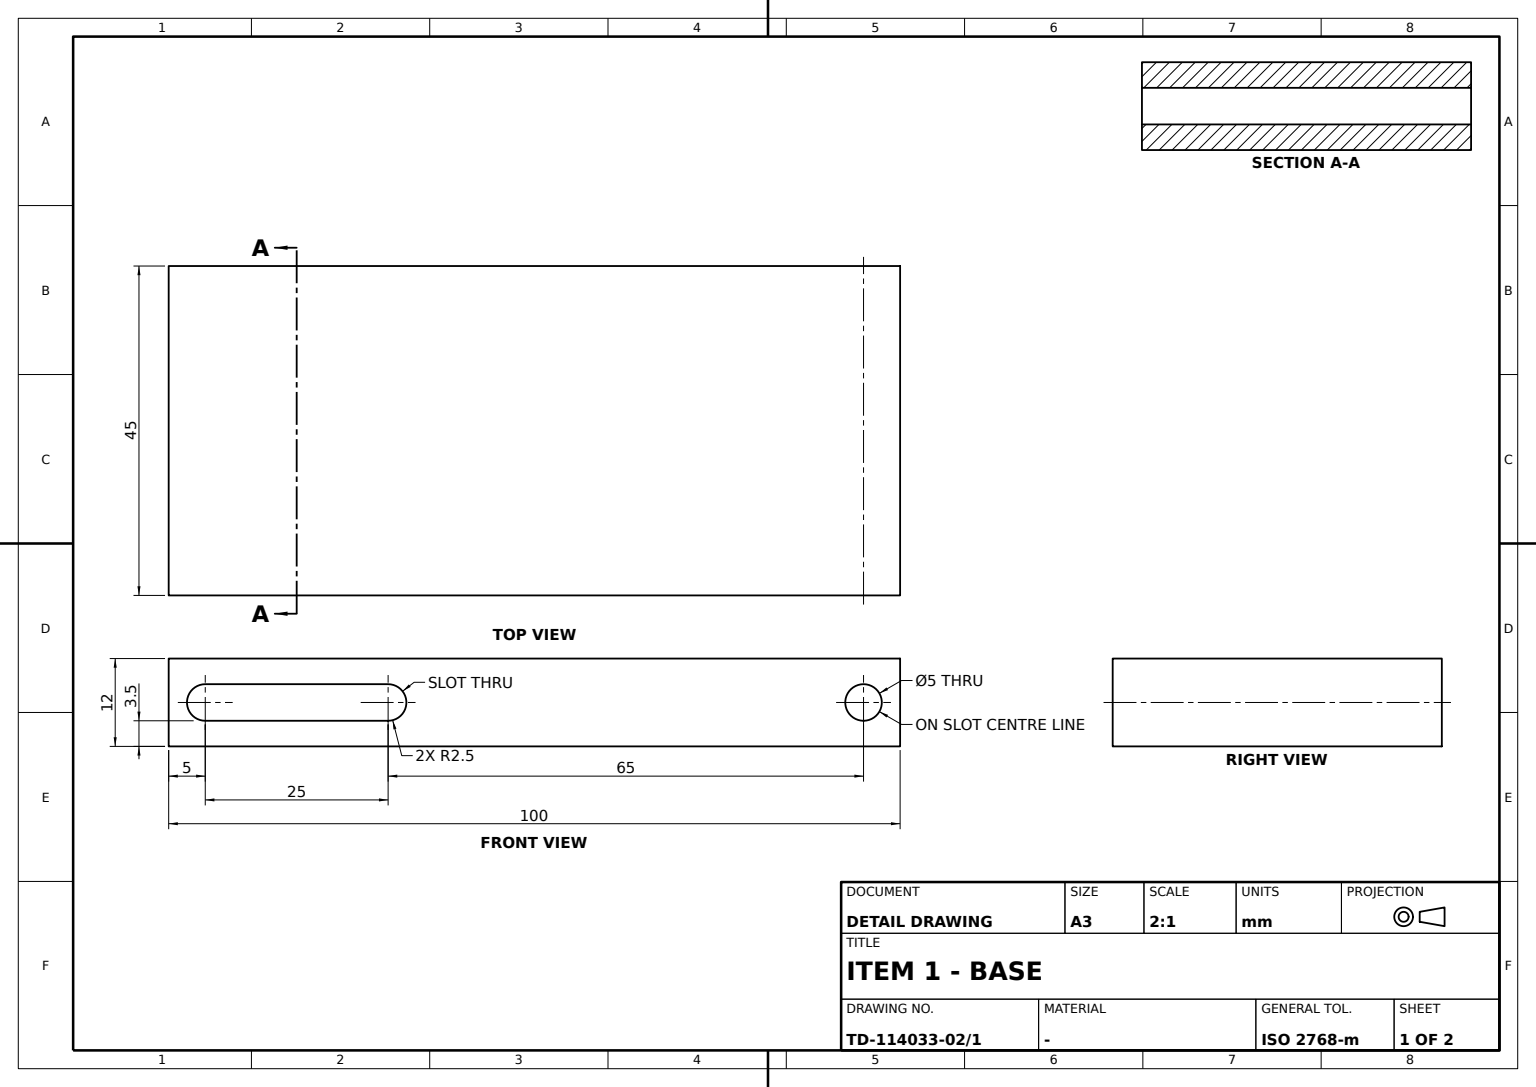
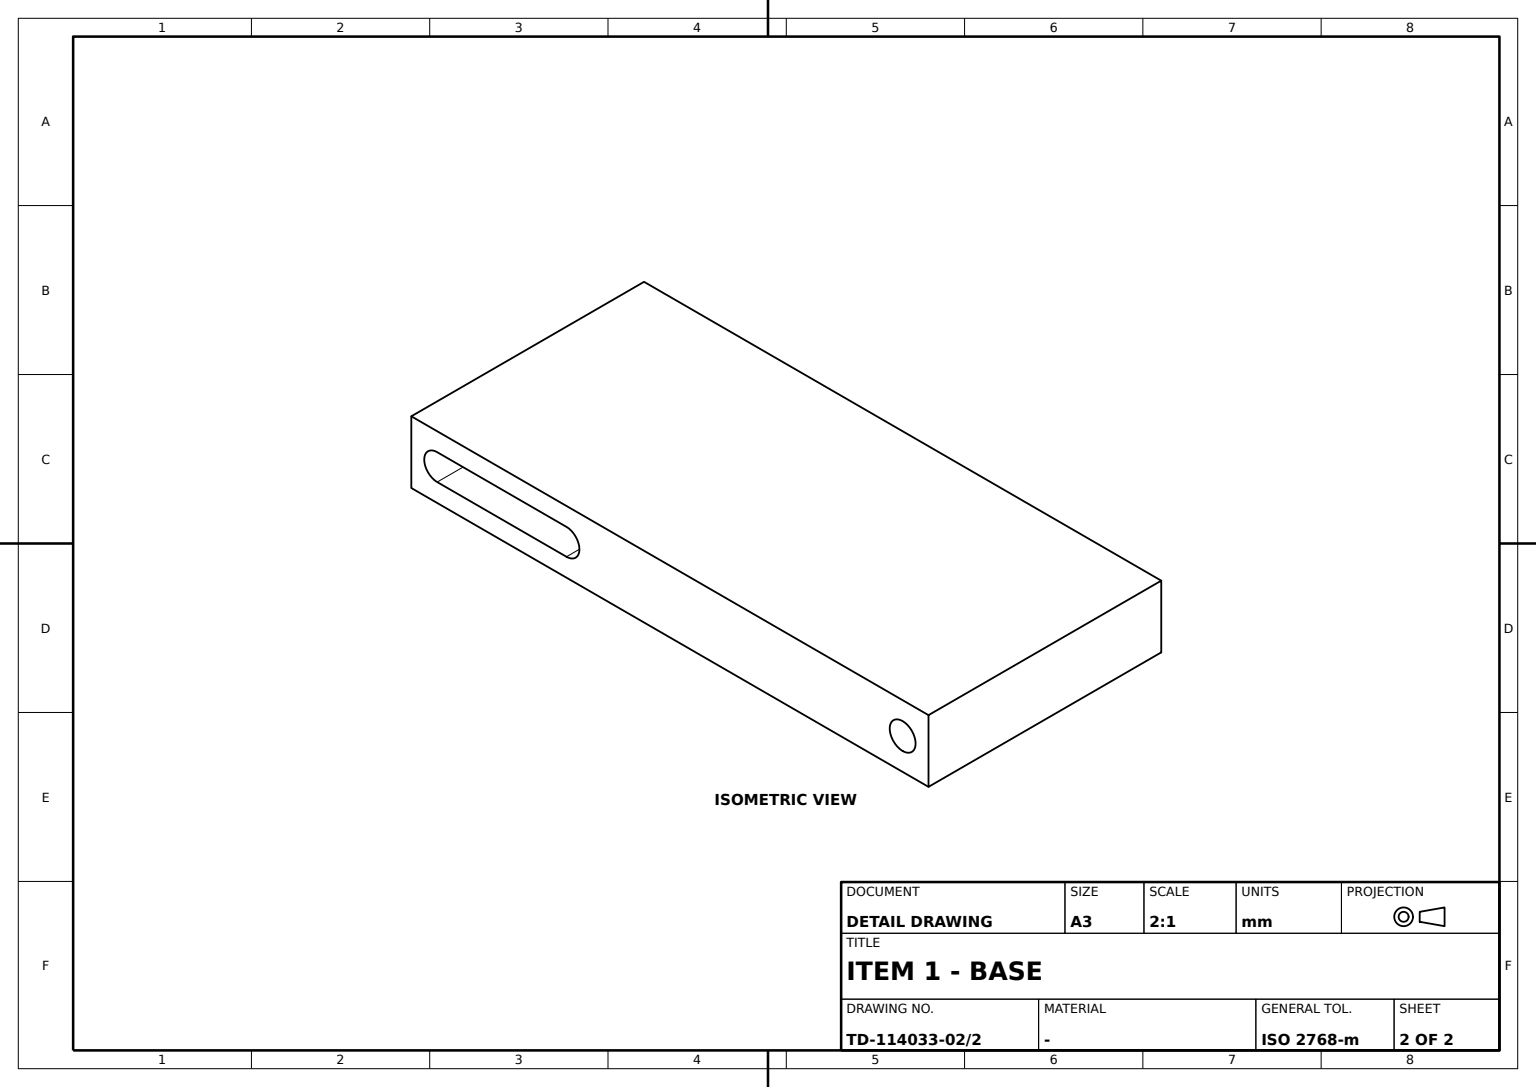
ISO-10303-21;
HEADER;
FILE_DESCRIPTION((''),'2;1');
FILE_NAME('','',(''),(''),'','','');
FILE_SCHEMA(('AUTOMOTIVE_DESIGN'));
ENDSEC;
DATA;
#1=APPLICATION_CONTEXT('');
#2=PRODUCT_CONTEXT('',#1,'mechanical');
#3=PRODUCT('','','',(#2));
#4=PRODUCT_DEFINITION_FORMATION('','',#3);
#5=PRODUCT_DEFINITION_CONTEXT('',#1,'design');
#6=PRODUCT_DEFINITION('','',#4,#5);
#7=PRODUCT_DEFINITION_SHAPE('','',#6);
#8=(LENGTH_UNIT()NAMED_UNIT(*)SI_UNIT(.MILLI.,.METRE.));
#9=(NAMED_UNIT(*)PLANE_ANGLE_UNIT()SI_UNIT($,.RADIAN.));
#10=(NAMED_UNIT(*)SI_UNIT($,.STERADIAN.)SOLID_ANGLE_UNIT());
#11=UNCERTAINTY_MEASURE_WITH_UNIT(LENGTH_MEASURE(0.005),#8,'distance_accuracy_value','');
#12=(GEOMETRIC_REPRESENTATION_CONTEXT(3)GLOBAL_UNCERTAINTY_ASSIGNED_CONTEXT((#11))GLOBAL_UNIT_ASSIGNED_CONTEXT((#8,#9,#10))REPRESENTATION_CONTEXT('',''));
#13=CARTESIAN_POINT('',(22.5,-20.,-2.5));
#14=VERTEX_POINT('',#13);
#15=CARTESIAN_POINT('',(22.5,-45.,-2.5));
#16=VERTEX_POINT('',#15);
#17=DIRECTION('',(0.,-1.,0.));
#18=VECTOR('',#17,1000.);
#19=LINE('',#13,#18);
#20=EDGE_CURVE('',#14,#16,#19,.T.);
#21=ORIENTED_EDGE('',*,*,#20,.F.);
#22=CARTESIAN_POINT('',(-22.5,-20.,-2.5));
#23=VERTEX_POINT('',#22);
#24=CARTESIAN_POINT('',(-0.66,-20.,-2.5));
#25=DIRECTION('',(1.,0.,0.));
#26=VECTOR('',#25,1000.);
#27=LINE('',#24,#26);
#28=EDGE_CURVE('',#14,#23,#27,.F.);
#29=ORIENTED_EDGE('',*,*,#28,.T.);
#30=CARTESIAN_POINT('',(-22.5,-45.,-2.5));
#31=VERTEX_POINT('',#30);
#32=LINE('',#22,#18);
#33=EDGE_CURVE('',#23,#31,#32,.T.);
#34=ORIENTED_EDGE('',*,*,#33,.T.);
#35=CARTESIAN_POINT('',(-0.66,-45.,-2.5));
#36=LINE('',#35,#26);
#37=EDGE_CURVE('',#16,#31,#36,.F.);
#38=ORIENTED_EDGE('',*,*,#37,.F.);
#39=EDGE_LOOP('',(#21,#29,#34,#38));
#40=FACE_BOUND('',#39,.T.);
#41=DIRECTION('',(0.,0.,-1.));
#42=AXIS2_PLACEMENT_3D('',#13,#41,#17);
#43=PLANE('',#42);
#44=ADVANCED_FACE('',(#40),#43,.F.);
#45=CARTESIAN_POINT('',(-22.5,50.,6.));
#46=VERTEX_POINT('',#45);
#47=CARTESIAN_POINT('',(-22.5,50.,-6.));
#48=VERTEX_POINT('',#47);
#49=CARTESIAN_POINT('',(-22.5,50.,0.));
#50=VECTOR('',#41,1000.);
#51=LINE('',#49,#50);
#52=EDGE_CURVE('',#46,#48,#51,.T.);
#53=ORIENTED_EDGE('',*,*,#52,.F.);
#54=CARTESIAN_POINT('',(22.5,50.,6.));
#55=VERTEX_POINT('',#54);
#56=CARTESIAN_POINT('',(0.,50.,6.));
#57=LINE('',#56,#26);
#58=EDGE_CURVE('',#46,#55,#57,.T.);
#59=ORIENTED_EDGE('',*,*,#58,.T.);
#60=CARTESIAN_POINT('',(22.5,50.,-6.));
#61=VERTEX_POINT('',#60);
#62=CARTESIAN_POINT('',(22.5,50.,0.));
#63=LINE('',#62,#50);
#64=EDGE_CURVE('',#55,#61,#63,.T.);
#65=ORIENTED_EDGE('',*,*,#64,.T.);
#66=CARTESIAN_POINT('',(0.,50.,-6.));
#67=LINE('',#66,#26);
#68=EDGE_CURVE('',#48,#61,#67,.T.);
#69=ORIENTED_EDGE('',*,*,#68,.F.);
#70=EDGE_LOOP('',(#53,#59,#65,#69));
#71=FACE_BOUND('',#70,.T.);
#72=AXIS2_PLACEMENT_3D('',#56,#17,#41);
#73=PLANE('',#72);
#74=ADVANCED_FACE('',(#71),#73,.F.);
#75=CARTESIAN_POINT('',(-22.5,-50.,6.));
#76=VERTEX_POINT('',#75);
#77=CARTESIAN_POINT('',(22.5,-50.,6.));
#78=VERTEX_POINT('',#77);
#79=CARTESIAN_POINT('',(0.,-50.,6.));
#80=LINE('',#79,#26);
#81=EDGE_CURVE('',#76,#78,#80,.T.);
#82=ORIENTED_EDGE('',*,*,#81,.F.);
#83=CARTESIAN_POINT('',(-22.5,-50.,-6.));
#84=VERTEX_POINT('',#83);
#85=CARTESIAN_POINT('',(-22.5,-50.,0.));
#86=DIRECTION('',(0.,0.,1.));
#87=VECTOR('',#86,1000.);
#88=LINE('',#85,#87);
#89=EDGE_CURVE('',#84,#76,#88,.T.);
#90=ORIENTED_EDGE('',*,*,#89,.F.);
#91=CARTESIAN_POINT('',(22.5,-50.,-6.));
#92=VERTEX_POINT('',#91);
#93=CARTESIAN_POINT('',(0.,-50.,-6.));
#94=LINE('',#93,#26);
#95=EDGE_CURVE('',#84,#92,#94,.T.);
#96=ORIENTED_EDGE('',*,*,#95,.T.);
#97=CARTESIAN_POINT('',(22.5,-50.,0.));
#98=LINE('',#97,#87);
#99=EDGE_CURVE('',#92,#78,#98,.T.);
#100=ORIENTED_EDGE('',*,*,#99,.T.);
#101=EDGE_LOOP('',(#82,#90,#96,#100));
#102=FACE_BOUND('',#101,.T.);
#103=DIRECTION('',(0.,1.,0.));
#104=AXIS2_PLACEMENT_3D('',#93,#103,#86);
#105=PLANE('',#104);
#106=ADVANCED_FACE('',(#102),#105,.F.);
#107=CARTESIAN_POINT('',(22.5,-45.,2.5));
#108=VERTEX_POINT('',#107);
#109=CARTESIAN_POINT('',(22.5,-45.,0.));
#110=AXIS2_PLACEMENT_3D('',#109,#25,#41);
#111=CIRCLE('',#110,2.5);
#112=EDGE_CURVE('',#108,#16,#111,.T.);
#113=ORIENTED_EDGE('',*,*,#112,.T.);
#114=ORIENTED_EDGE('',*,*,#37,.T.);
#115=CARTESIAN_POINT('',(-22.5,-45.,2.5));
#116=VERTEX_POINT('',#115);
#117=CARTESIAN_POINT('',(-22.5,-45.,0.));
#118=AXIS2_PLACEMENT_3D('',#117,#25,#41);
#119=CIRCLE('',#118,2.5);
#120=EDGE_CURVE('',#116,#31,#119,.T.);
#121=ORIENTED_EDGE('',*,*,#120,.F.);
#122=CARTESIAN_POINT('',(-0.66,-45.,2.5));
#123=LINE('',#122,#26);
#124=EDGE_CURVE('',#108,#116,#123,.F.);
#125=ORIENTED_EDGE('',*,*,#124,.F.);
#126=EDGE_LOOP('',(#113,#114,#121,#125));
#127=FACE_BOUND('',#126,.T.);
#128=CARTESIAN_POINT('',(-0.66,-45.,0.));
#129=AXIS2_PLACEMENT_3D('',#128,#25,#103);
#130=CYLINDRICAL_SURFACE('',#129,2.5);
#131=ADVANCED_FACE('',(#127),#130,.F.);
#132=CARTESIAN_POINT('',(22.5,-20.,2.5));
#133=VERTEX_POINT('',#132);
#134=VECTOR('',#103,1000.);
#135=LINE('',#107,#134);
#136=EDGE_CURVE('',#108,#133,#135,.T.);
#137=ORIENTED_EDGE('',*,*,#136,.F.);
#138=ORIENTED_EDGE('',*,*,#124,.T.);
#139=CARTESIAN_POINT('',(-22.5,-20.,2.5));
#140=VERTEX_POINT('',#139);
#141=LINE('',#115,#134);
#142=EDGE_CURVE('',#116,#140,#141,.T.);
#143=ORIENTED_EDGE('',*,*,#142,.T.);
#144=CARTESIAN_POINT('',(-0.66,-20.,2.5));
#145=LINE('',#144,#26);
#146=EDGE_CURVE('',#133,#140,#145,.F.);
#147=ORIENTED_EDGE('',*,*,#146,.F.);
#148=EDGE_LOOP('',(#137,#138,#143,#147));
#149=FACE_BOUND('',#148,.T.);
#150=AXIS2_PLACEMENT_3D('',#107,#86,#103);
#151=PLANE('',#150);
#152=ADVANCED_FACE('',(#149),#151,.F.);
#153=CARTESIAN_POINT('',(22.5,0.,-6.));
#154=LINE('',#153,#18);
#155=EDGE_CURVE('',#61,#92,#154,.T.);
#156=ORIENTED_EDGE('',*,*,#155,.T.);
#157=ORIENTED_EDGE('',*,*,#95,.F.);
#158=CARTESIAN_POINT('',(-22.5,0.,-6.));
#159=LINE('',#158,#18);
#160=EDGE_CURVE('',#48,#84,#159,.T.);
#161=ORIENTED_EDGE('',*,*,#160,.F.);
#162=ORIENTED_EDGE('',*,*,#68,.T.);
#163=EDGE_LOOP('',(#156,#157,#161,#162));
#164=FACE_BOUND('',#163,.T.);
#165=AXIS2_PLACEMENT_3D('',#66,#86,#17);
#166=PLANE('',#165);
#167=ADVANCED_FACE('',(#164),#166,.F.);
#168=ORIENTED_EDGE('',*,*,#99,.F.);
#169=ORIENTED_EDGE('',*,*,#155,.F.);
#170=ORIENTED_EDGE('',*,*,#64,.F.);
#171=CARTESIAN_POINT('',(22.5,0.,6.));
#172=LINE('',#171,#134);
#173=EDGE_CURVE('',#78,#55,#172,.T.);
#174=ORIENTED_EDGE('',*,*,#173,.F.);
#175=EDGE_LOOP('',(#168,#169,#170,#174));
#176=FACE_BOUND('',#175,.T.);
#177=ORIENTED_EDGE('',*,*,#20,.T.);
#178=ORIENTED_EDGE('',*,*,#112,.F.);
#179=ORIENTED_EDGE('',*,*,#136,.T.);
#180=CARTESIAN_POINT('',(22.5,-20.,0.));
#181=AXIS2_PLACEMENT_3D('',#180,#25,#41);
#182=CIRCLE('',#181,2.5);
#183=EDGE_CURVE('',#14,#133,#182,.T.);
#184=ORIENTED_EDGE('',*,*,#183,.F.);
#185=EDGE_LOOP('',(#177,#178,#179,#184));
#186=FACE_BOUND('',#185,.T.);
#187=CARTESIAN_POINT('',(22.5,45.,-2.5));
#188=VERTEX_POINT('',#187);
#189=CARTESIAN_POINT('',(22.5,45.,0.));
#190=AXIS2_PLACEMENT_3D('',#189,#25,#41);
#191=CIRCLE('',#190,2.5);
#192=EDGE_CURVE('',#188,#188,#191,.T.);
#193=ORIENTED_EDGE('',*,*,#192,.F.);
#194=EDGE_LOOP('',(#193));
#195=FACE_BOUND('',#194,.T.);
#196=CARTESIAN_POINT('',(22.5,0.,0.));
#197=AXIS2_PLACEMENT_3D('',#196,#25,#103);
#198=PLANE('',#197);
#199=ADVANCED_FACE('',(#176,#186,#195),#198,.T.);
#200=ORIENTED_EDGE('',*,*,#160,.T.);
#201=ORIENTED_EDGE('',*,*,#89,.T.);
#202=CARTESIAN_POINT('',(-22.5,0.,6.));
#203=LINE('',#202,#134);
#204=EDGE_CURVE('',#76,#46,#203,.T.);
#205=ORIENTED_EDGE('',*,*,#204,.T.);
#206=ORIENTED_EDGE('',*,*,#52,.T.);
#207=EDGE_LOOP('',(#200,#201,#205,#206));
#208=FACE_BOUND('',#207,.T.);
#209=CARTESIAN_POINT('',(-22.5,45.,-2.5));
#210=VERTEX_POINT('',#209);
#211=CARTESIAN_POINT('',(-22.5,45.,0.));
#212=AXIS2_PLACEMENT_3D('',#211,#25,#41);
#213=CIRCLE('',#212,2.5);
#214=EDGE_CURVE('',#210,#210,#213,.T.);
#215=ORIENTED_EDGE('',*,*,#214,.T.);
#216=EDGE_LOOP('',(#215));
#217=FACE_BOUND('',#216,.T.);
#218=ORIENTED_EDGE('',*,*,#33,.F.);
#219=CARTESIAN_POINT('',(-22.5,-20.,0.));
#220=AXIS2_PLACEMENT_3D('',#219,#25,#41);
#221=CIRCLE('',#220,2.5);
#222=EDGE_CURVE('',#23,#140,#221,.T.);
#223=ORIENTED_EDGE('',*,*,#222,.T.);
#224=ORIENTED_EDGE('',*,*,#142,.F.);
#225=ORIENTED_EDGE('',*,*,#120,.T.);
#226=EDGE_LOOP('',(#218,#223,#224,#225));
#227=FACE_BOUND('',#226,.T.);
#228=CARTESIAN_POINT('',(-22.5,0.,0.));
#229=AXIS2_PLACEMENT_3D('',#228,#25,#103);
#230=PLANE('',#229);
#231=ADVANCED_FACE('',(#208,#217,#227),#230,.F.);
#232=ORIENTED_EDGE('',*,*,#28,.F.);
#233=ORIENTED_EDGE('',*,*,#183,.T.);
#234=ORIENTED_EDGE('',*,*,#146,.T.);
#235=ORIENTED_EDGE('',*,*,#222,.F.);
#236=EDGE_LOOP('',(#232,#233,#234,#235));
#237=FACE_BOUND('',#236,.T.);
#238=CARTESIAN_POINT('',(-0.66,-20.,0.));
#239=AXIS2_PLACEMENT_3D('',#238,#25,#103);
#240=CYLINDRICAL_SURFACE('',#239,2.5);
#241=ADVANCED_FACE('',(#237),#240,.F.);
#242=ORIENTED_EDGE('',*,*,#81,.T.);
#243=ORIENTED_EDGE('',*,*,#173,.T.);
#244=ORIENTED_EDGE('',*,*,#58,.F.);
#245=ORIENTED_EDGE('',*,*,#204,.F.);
#246=EDGE_LOOP('',(#242,#243,#244,#245));
#247=FACE_BOUND('',#246,.T.);
#248=AXIS2_PLACEMENT_3D('',#79,#41,#103);
#249=PLANE('',#248);
#250=ADVANCED_FACE('',(#247),#249,.F.);
#251=ORIENTED_EDGE('',*,*,#192,.T.);
#252=EDGE_LOOP('',(#251));
#253=FACE_BOUND('',#252,.T.);
#254=ORIENTED_EDGE('',*,*,#214,.F.);
#255=EDGE_LOOP('',(#254));
#256=FACE_BOUND('',#255,.T.);
#257=CARTESIAN_POINT('',(-0.66,45.,0.));
#258=AXIS2_PLACEMENT_3D('',#257,#25,#103);
#259=CYLINDRICAL_SURFACE('',#258,2.5);
#260=ADVANCED_FACE('',(#253,#256),#259,.F.);
#261=CLOSED_SHELL('',(#44,#74,#106,#131,#152,#167,#199,#231,#241,#250,#260));
#262=MANIFOLD_SOLID_BREP('',#261);
#263=ADVANCED_BREP_SHAPE_REPRESENTATION('',(#262),#12);
#264=SHAPE_DEFINITION_REPRESENTATION(#7,#263);
ENDSEC;
END-ISO-10303-21;
